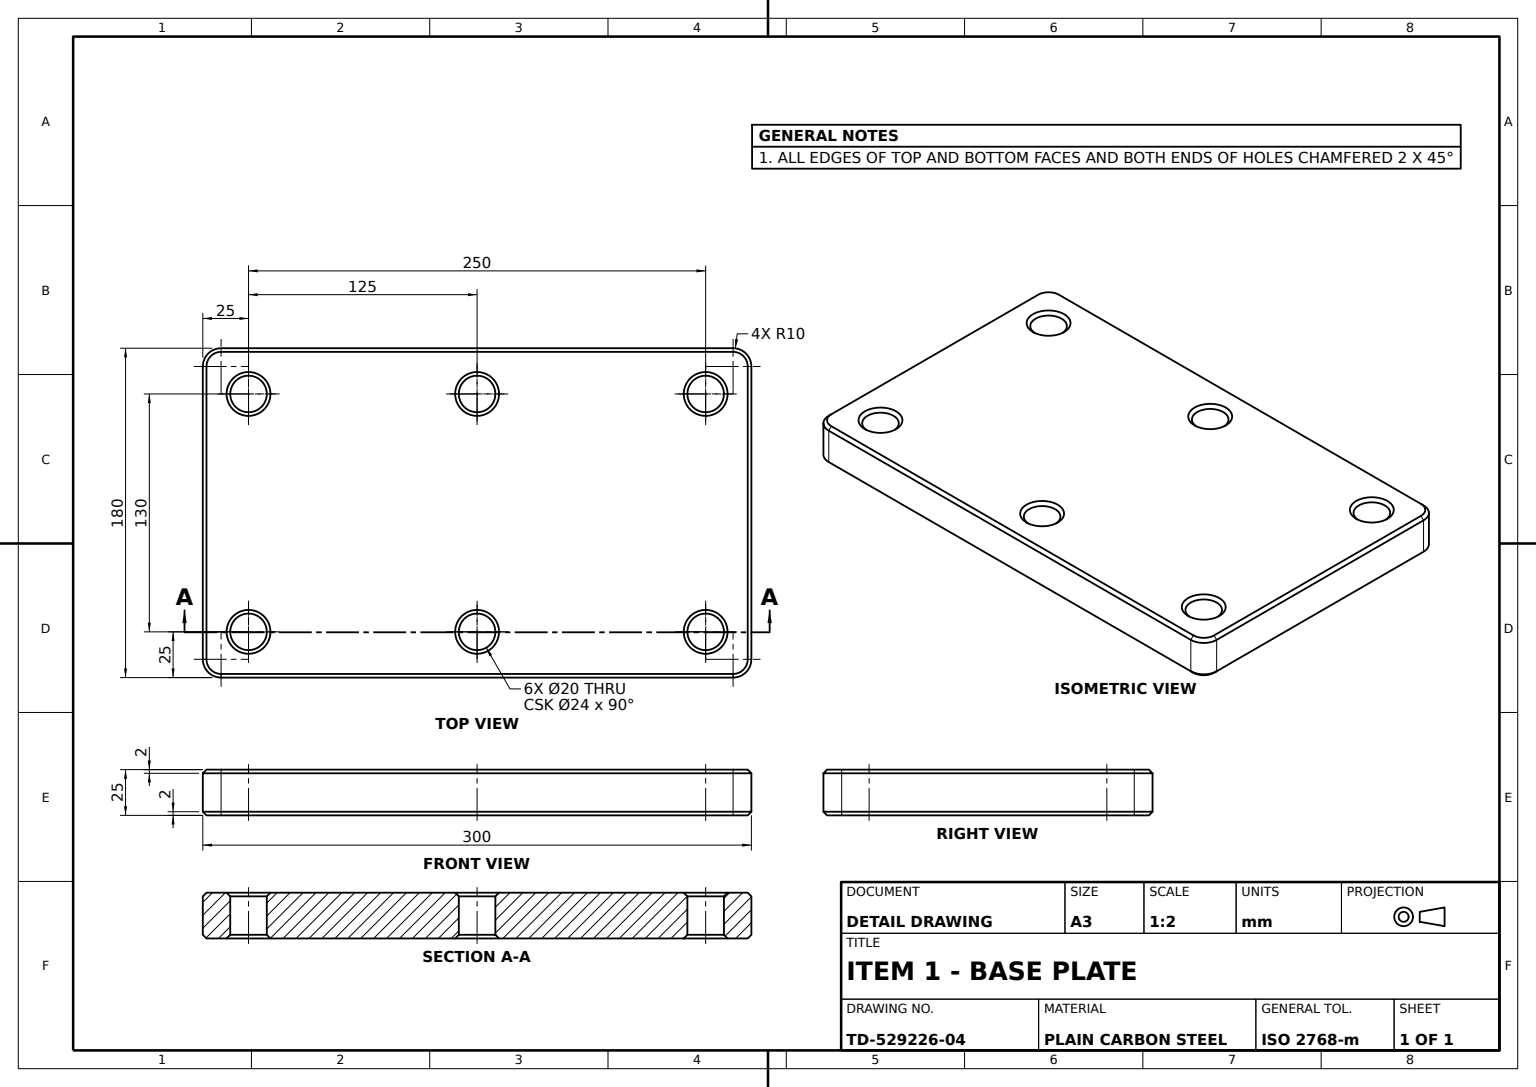
ISO-10303-21;
HEADER;
FILE_DESCRIPTION((''),'2;1');
FILE_NAME('','',(''),(''),'','','');
FILE_SCHEMA(('AUTOMOTIVE_DESIGN'));
ENDSEC;
DATA;
#1=APPLICATION_CONTEXT('');
#2=PRODUCT_CONTEXT('',#1,'mechanical');
#3=PRODUCT('','','',(#2));
#4=PRODUCT_DEFINITION_FORMATION('','',#3);
#5=PRODUCT_DEFINITION_CONTEXT('',#1,'design');
#6=PRODUCT_DEFINITION('','',#4,#5);
#7=PRODUCT_DEFINITION_SHAPE('','',#6);
#8=(LENGTH_UNIT()NAMED_UNIT(*)SI_UNIT(.MILLI.,.METRE.));
#9=(NAMED_UNIT(*)PLANE_ANGLE_UNIT()SI_UNIT($,.RADIAN.));
#10=(NAMED_UNIT(*)SI_UNIT($,.STERADIAN.)SOLID_ANGLE_UNIT());
#11=UNCERTAINTY_MEASURE_WITH_UNIT(LENGTH_MEASURE(1.E-05),#8,'distance_accuracy_value','');
#12=(GEOMETRIC_REPRESENTATION_CONTEXT(3)GLOBAL_UNCERTAINTY_ASSIGNED_CONTEXT((#11))GLOBAL_UNIT_ASSIGNED_CONTEXT((#8,#9,#10))REPRESENTATION_CONTEXT('',''));
#13=CARTESIAN_POINT('',(-150.,23.,-80.));
#14=VERTEX_POINT('',#13);
#15=CARTESIAN_POINT('',(-140.,23.,-90.));
#16=VERTEX_POINT('',#15);
#17=CARTESIAN_POINT('',(-140.,23.,-80.));
#18=DIRECTION('',(0.,-1.,0.));
#19=DIRECTION('',(0.,0.,-1.));
#20=AXIS2_PLACEMENT_3D('',#17,#18,#19);
#21=CIRCLE('',#20,10.);
#22=EDGE_CURVE('',#14,#16,#21,.T.);
#23=ORIENTED_EDGE('',*,*,#22,.T.);
#24=CARTESIAN_POINT('',(-140.,2.,-90.));
#25=VERTEX_POINT('',#24);
#26=CARTESIAN_POINT('',(-140.,25.,-90.));
#27=VECTOR('',#18,1000.);
#28=LINE('',#26,#27);
#29=EDGE_CURVE('',#16,#25,#28,.T.);
#30=ORIENTED_EDGE('',*,*,#29,.T.);
#31=CARTESIAN_POINT('',(-150.,2.,-80.));
#32=VERTEX_POINT('',#31);
#33=CARTESIAN_POINT('',(-140.,2.,-80.));
#34=DIRECTION('',(0.,1.,0.));
#35=AXIS2_PLACEMENT_3D('',#33,#34,#19);
#36=CIRCLE('',#35,10.);
#37=EDGE_CURVE('',#25,#32,#36,.T.);
#38=ORIENTED_EDGE('',*,*,#37,.T.);
#39=CARTESIAN_POINT('',(-150.,25.,-80.));
#40=LINE('',#39,#27);
#41=EDGE_CURVE('',#14,#32,#40,.T.);
#42=ORIENTED_EDGE('',*,*,#41,.F.);
#43=EDGE_LOOP('',(#23,#30,#38,#42));
#44=FACE_OUTER_BOUND('',#43,.T.);
#45=CARTESIAN_POINT('',(-140.,25.,-80.));
#46=AXIS2_PLACEMENT_3D('',#45,#18,#19);
#47=CYLINDRICAL_SURFACE('',#46,10.);
#48=ADVANCED_FACE('',(#44),#47,.T.);
#49=CARTESIAN_POINT('',(0.,2.,-55.));
#50=VERTEX_POINT('',#49);
#51=CARTESIAN_POINT('',(0.,2.,-75.));
#52=VERTEX_POINT('',#51);
#53=CARTESIAN_POINT('',(0.,2.,-65.));
#54=AXIS2_PLACEMENT_3D('',#53,#18,#19);
#55=CIRCLE('',#54,10.);
#56=EDGE_CURVE('',#50,#52,#55,.T.);
#57=ORIENTED_EDGE('',*,*,#56,.F.);
#58=CARTESIAN_POINT('',(0.,0.,-53.));
#59=VERTEX_POINT('',#58);
#60=DIRECTION('',(0.,-0.707106781,0.707106781));
#61=VECTOR('',#60,1000.);
#62=LINE('',#58,#61);
#63=EDGE_CURVE('',#50,#59,#62,.T.);
#64=ORIENTED_EDGE('',*,*,#63,.T.);
#65=CARTESIAN_POINT('',(0.,0.,-77.));
#66=VERTEX_POINT('',#65);
#67=CARTESIAN_POINT('',(0.,0.,-65.));
#68=AXIS2_PLACEMENT_3D('',#67,#34,#19);
#69=CIRCLE('',#68,12.);
#70=EDGE_CURVE('',#66,#59,#69,.T.);
#71=ORIENTED_EDGE('',*,*,#70,.F.);
#72=DIRECTION('',(0.,-0.707106781,-0.707106781));
#73=VECTOR('',#72,1000.);
#74=LINE('',#65,#73);
#75=EDGE_CURVE('',#52,#66,#74,.T.);
#76=ORIENTED_EDGE('',*,*,#75,.F.);
#77=EDGE_LOOP('',(#57,#64,#71,#76));
#78=FACE_OUTER_BOUND('',#77,.T.);
#79=AXIS2_PLACEMENT_3D('',#67,#18,#19);
#80=CONICAL_SURFACE('',#79,12.,0.785398163);
#81=ADVANCED_FACE('',(#78),#80,.F.);
#82=CARTESIAN_POINT('',(-140.,23.,90.));
#83=VERTEX_POINT('',#82);
#84=CARTESIAN_POINT('',(-150.,23.,80.));
#85=VERTEX_POINT('',#84);
#86=CARTESIAN_POINT('',(-140.,23.,80.));
#87=AXIS2_PLACEMENT_3D('',#86,#18,#19);
#88=CIRCLE('',#87,10.);
#89=EDGE_CURVE('',#83,#85,#88,.T.);
#90=ORIENTED_EDGE('',*,*,#89,.F.);
#91=CARTESIAN_POINT('',(-140.,25.,88.));
#92=VERTEX_POINT('',#91);
#93=LINE('',#91,#61);
#94=EDGE_CURVE('',#92,#83,#93,.T.);
#95=ORIENTED_EDGE('',*,*,#94,.F.);
#96=CARTESIAN_POINT('',(-148.,25.,80.));
#97=VERTEX_POINT('',#96);
#98=CARTESIAN_POINT('',(-140.,25.,80.));
#99=AXIS2_PLACEMENT_3D('',#98,#34,#19);
#100=CIRCLE('',#99,8.);
#101=EDGE_CURVE('',#97,#92,#100,.T.);
#102=ORIENTED_EDGE('',*,*,#101,.F.);
#103=DIRECTION('',(-0.707106781,-0.707106781,0.));
#104=VECTOR('',#103,1000.);
#105=LINE('',#96,#104);
#106=EDGE_CURVE('',#97,#85,#105,.T.);
#107=ORIENTED_EDGE('',*,*,#106,.T.);
#108=EDGE_LOOP('',(#90,#95,#102,#107));
#109=FACE_OUTER_BOUND('',#108,.T.);
#110=AXIS2_PLACEMENT_3D('',#98,#18,#19);
#111=CONICAL_SURFACE('',#110,8.,0.785398163);
#112=ADVANCED_FACE('',(#109),#111,.T.);
#113=CARTESIAN_POINT('',(0.,23.,-75.));
#114=VERTEX_POINT('',#113);
#115=CARTESIAN_POINT('',(0.,23.,-55.));
#116=VERTEX_POINT('',#115);
#117=CARTESIAN_POINT('',(0.,23.,-65.));
#118=AXIS2_PLACEMENT_3D('',#117,#34,#19);
#119=CIRCLE('',#118,10.);
#120=EDGE_CURVE('',#114,#116,#119,.T.);
#121=ORIENTED_EDGE('',*,*,#120,.F.);
#122=CARTESIAN_POINT('',(0.,25.,-77.));
#123=VERTEX_POINT('',#122);
#124=DIRECTION('',(0.,0.707106781,-0.707106781));
#125=VECTOR('',#124,1000.);
#126=LINE('',#113,#125);
#127=EDGE_CURVE('',#114,#123,#126,.T.);
#128=ORIENTED_EDGE('',*,*,#127,.T.);
#129=CARTESIAN_POINT('',(0.,25.,-53.));
#130=VERTEX_POINT('',#129);
#131=CARTESIAN_POINT('',(0.,25.,-65.));
#132=AXIS2_PLACEMENT_3D('',#131,#18,#19);
#133=CIRCLE('',#132,12.);
#134=EDGE_CURVE('',#130,#123,#133,.T.);
#135=ORIENTED_EDGE('',*,*,#134,.F.);
#136=DIRECTION('',(0.,0.707106781,0.707106781));
#137=VECTOR('',#136,1000.);
#138=LINE('',#115,#137);
#139=EDGE_CURVE('',#116,#130,#138,.T.);
#140=ORIENTED_EDGE('',*,*,#139,.F.);
#141=EDGE_LOOP('',(#121,#128,#135,#140));
#142=FACE_OUTER_BOUND('',#141,.T.);
#143=DIRECTION('',(0.,0.,1.));
#144=AXIS2_PLACEMENT_3D('',#117,#34,#143);
#145=CONICAL_SURFACE('',#144,10.,0.785398163);
#146=ADVANCED_FACE('',(#142),#145,.F.);
#147=CARTESIAN_POINT('',(-125.,2.,55.));
#148=VERTEX_POINT('',#147);
#149=CARTESIAN_POINT('',(-125.,0.,53.));
#150=VERTEX_POINT('',#149);
#151=LINE('',#149,#73);
#152=EDGE_CURVE('',#148,#150,#151,.T.);
#153=ORIENTED_EDGE('',*,*,#152,.T.);
#154=CARTESIAN_POINT('',(-125.,0.,77.));
#155=VERTEX_POINT('',#154);
#156=CARTESIAN_POINT('',(-125.,0.,65.));
#157=AXIS2_PLACEMENT_3D('',#156,#34,#19);
#158=CIRCLE('',#157,12.);
#159=EDGE_CURVE('',#155,#150,#158,.T.);
#160=ORIENTED_EDGE('',*,*,#159,.F.);
#161=CARTESIAN_POINT('',(-125.,2.,75.));
#162=VERTEX_POINT('',#161);
#163=LINE('',#154,#61);
#164=EDGE_CURVE('',#162,#155,#163,.T.);
#165=ORIENTED_EDGE('',*,*,#164,.F.);
#166=CARTESIAN_POINT('',(-125.,2.,65.));
#167=AXIS2_PLACEMENT_3D('',#166,#18,#19);
#168=CIRCLE('',#167,10.);
#169=EDGE_CURVE('',#148,#162,#168,.T.);
#170=ORIENTED_EDGE('',*,*,#169,.F.);
#171=EDGE_LOOP('',(#153,#160,#165,#170));
#172=FACE_OUTER_BOUND('',#171,.T.);
#173=AXIS2_PLACEMENT_3D('',#156,#18,#19);
#174=CONICAL_SURFACE('',#173,12.,0.785398163);
#175=ADVANCED_FACE('',(#172),#174,.F.);
#176=CARTESIAN_POINT('',(-125.,23.,55.));
#177=VERTEX_POINT('',#176);
#178=CARTESIAN_POINT('',(-125.,25.,55.));
#179=LINE('',#178,#27);
#180=EDGE_CURVE('',#177,#148,#179,.T.);
#181=ORIENTED_EDGE('',*,*,#180,.T.);
#182=ORIENTED_EDGE('',*,*,#169,.T.);
#183=CARTESIAN_POINT('',(-125.,23.,75.));
#184=VERTEX_POINT('',#183);
#185=CARTESIAN_POINT('',(-125.,25.,75.));
#186=LINE('',#185,#27);
#187=EDGE_CURVE('',#184,#162,#186,.T.);
#188=ORIENTED_EDGE('',*,*,#187,.F.);
#189=CARTESIAN_POINT('',(-125.,23.,65.));
#190=AXIS2_PLACEMENT_3D('',#189,#34,#19);
#191=CIRCLE('',#190,10.);
#192=EDGE_CURVE('',#184,#177,#191,.T.);
#193=ORIENTED_EDGE('',*,*,#192,.T.);
#194=EDGE_LOOP('',(#181,#182,#188,#193));
#195=FACE_OUTER_BOUND('',#194,.T.);
#196=CARTESIAN_POINT('',(-125.,25.,65.));
#197=AXIS2_PLACEMENT_3D('',#196,#18,#19);
#198=CYLINDRICAL_SURFACE('',#197,10.);
#199=ADVANCED_FACE('',(#195),#198,.F.);
#200=CARTESIAN_POINT('',(150.,2.,80.));
#201=VERTEX_POINT('',#200);
#202=CARTESIAN_POINT('',(150.,2.,-80.));
#203=VERTEX_POINT('',#202);
#204=VECTOR('',#19,1000.);
#205=LINE('',#202,#204);
#206=EDGE_CURVE('',#201,#203,#205,.T.);
#207=ORIENTED_EDGE('',*,*,#206,.F.);
#208=CARTESIAN_POINT('',(148.,0.,80.));
#209=VERTEX_POINT('',#208);
#210=LINE('',#200,#104);
#211=EDGE_CURVE('',#201,#209,#210,.T.);
#212=ORIENTED_EDGE('',*,*,#211,.T.);
#213=CARTESIAN_POINT('',(148.,0.,-80.));
#214=VERTEX_POINT('',#213);
#215=VECTOR('',#143,1000.);
#216=LINE('',#208,#215);
#217=EDGE_CURVE('',#214,#209,#216,.T.);
#218=ORIENTED_EDGE('',*,*,#217,.F.);
#219=LINE('',#202,#104);
#220=EDGE_CURVE('',#203,#214,#219,.T.);
#221=ORIENTED_EDGE('',*,*,#220,.F.);
#222=EDGE_LOOP('',(#207,#212,#218,#221));
#223=FACE_OUTER_BOUND('',#222,.T.);
#224=DIRECTION('',(0.707106781,-0.707106781,0.));
#225=AXIS2_PLACEMENT_3D('',#202,#224,#143);
#226=PLANE('',#225);
#227=ADVANCED_FACE('',(#223),#226,.T.);
#228=CARTESIAN_POINT('',(140.,0.,-88.));
#229=VERTEX_POINT('',#228);
#230=CARTESIAN_POINT('',(140.,0.,-80.));
#231=AXIS2_PLACEMENT_3D('',#230,#18,#19);
#232=CIRCLE('',#231,8.);
#233=EDGE_CURVE('',#229,#214,#232,.T.);
#234=ORIENTED_EDGE('',*,*,#233,.F.);
#235=CARTESIAN_POINT('',(140.,2.,-90.));
#236=VERTEX_POINT('',#235);
#237=LINE('',#235,#61);
#238=EDGE_CURVE('',#236,#229,#237,.T.);
#239=ORIENTED_EDGE('',*,*,#238,.F.);
#240=CARTESIAN_POINT('',(140.,2.,-80.));
#241=AXIS2_PLACEMENT_3D('',#240,#34,#19);
#242=CIRCLE('',#241,10.);
#243=EDGE_CURVE('',#203,#236,#242,.T.);
#244=ORIENTED_EDGE('',*,*,#243,.F.);
#245=ORIENTED_EDGE('',*,*,#220,.T.);
#246=EDGE_LOOP('',(#234,#239,#244,#245));
#247=FACE_OUTER_BOUND('',#246,.T.);
#248=AXIS2_PLACEMENT_3D('',#240,#34,#143);
#249=CONICAL_SURFACE('',#248,10.,0.785398163);
#250=ADVANCED_FACE('',(#247),#249,.T.);
#251=CARTESIAN_POINT('',(-140.,0.,88.));
#252=VERTEX_POINT('',#251);
#253=CARTESIAN_POINT('',(-140.,2.,90.));
#254=VERTEX_POINT('',#253);
#255=LINE('',#251,#137);
#256=EDGE_CURVE('',#252,#254,#255,.T.);
#257=ORIENTED_EDGE('',*,*,#256,.T.);
#258=CARTESIAN_POINT('',(-150.,2.,80.));
#259=VERTEX_POINT('',#258);
#260=CARTESIAN_POINT('',(-140.,2.,80.));
#261=AXIS2_PLACEMENT_3D('',#260,#34,#19);
#262=CIRCLE('',#261,10.);
#263=EDGE_CURVE('',#259,#254,#262,.T.);
#264=ORIENTED_EDGE('',*,*,#263,.F.);
#265=CARTESIAN_POINT('',(-148.,0.,80.));
#266=VERTEX_POINT('',#265);
#267=DIRECTION('',(-0.707106781,0.707106781,0.));
#268=VECTOR('',#267,1000.);
#269=LINE('',#265,#268);
#270=EDGE_CURVE('',#266,#259,#269,.T.);
#271=ORIENTED_EDGE('',*,*,#270,.F.);
#272=CARTESIAN_POINT('',(-140.,0.,80.));
#273=AXIS2_PLACEMENT_3D('',#272,#18,#19);
#274=CIRCLE('',#273,8.);
#275=EDGE_CURVE('',#252,#266,#274,.T.);
#276=ORIENTED_EDGE('',*,*,#275,.F.);
#277=EDGE_LOOP('',(#257,#264,#271,#276));
#278=FACE_OUTER_BOUND('',#277,.T.);
#279=AXIS2_PLACEMENT_3D('',#260,#34,#143);
#280=CONICAL_SURFACE('',#279,10.,0.785398163);
#281=ADVANCED_FACE('',(#278),#280,.T.);
#282=CARTESIAN_POINT('',(0.,2.,75.));
#283=VERTEX_POINT('',#282);
#284=CARTESIAN_POINT('',(0.,0.,77.));
#285=VERTEX_POINT('',#284);
#286=LINE('',#284,#61);
#287=EDGE_CURVE('',#283,#285,#286,.T.);
#288=ORIENTED_EDGE('',*,*,#287,.T.);
#289=CARTESIAN_POINT('',(0.,0.,53.));
#290=VERTEX_POINT('',#289);
#291=CARTESIAN_POINT('',(0.,0.,65.));
#292=AXIS2_PLACEMENT_3D('',#291,#34,#19);
#293=CIRCLE('',#292,12.);
#294=EDGE_CURVE('',#290,#285,#293,.T.);
#295=ORIENTED_EDGE('',*,*,#294,.F.);
#296=CARTESIAN_POINT('',(0.,2.,55.));
#297=VERTEX_POINT('',#296);
#298=LINE('',#289,#73);
#299=EDGE_CURVE('',#297,#290,#298,.T.);
#300=ORIENTED_EDGE('',*,*,#299,.F.);
#301=CARTESIAN_POINT('',(0.,2.,65.));
#302=AXIS2_PLACEMENT_3D('',#301,#18,#19);
#303=CIRCLE('',#302,10.);
#304=EDGE_CURVE('',#283,#297,#303,.T.);
#305=ORIENTED_EDGE('',*,*,#304,.F.);
#306=EDGE_LOOP('',(#288,#295,#300,#305));
#307=FACE_OUTER_BOUND('',#306,.T.);
#308=AXIS2_PLACEMENT_3D('',#291,#18,#19);
#309=CONICAL_SURFACE('',#308,12.,0.785398163);
#310=ADVANCED_FACE('',(#307),#309,.F.);
#311=CARTESIAN_POINT('',(125.,2.,55.));
#312=VERTEX_POINT('',#311);
#313=CARTESIAN_POINT('',(125.,2.,75.));
#314=VERTEX_POINT('',#313);
#315=CARTESIAN_POINT('',(125.,2.,65.));
#316=AXIS2_PLACEMENT_3D('',#315,#18,#19);
#317=CIRCLE('',#316,10.);
#318=EDGE_CURVE('',#312,#314,#317,.T.);
#319=ORIENTED_EDGE('',*,*,#318,.T.);
#320=CARTESIAN_POINT('',(125.,23.,75.));
#321=VERTEX_POINT('',#320);
#322=CARTESIAN_POINT('',(125.,25.,75.));
#323=LINE('',#322,#27);
#324=EDGE_CURVE('',#321,#314,#323,.T.);
#325=ORIENTED_EDGE('',*,*,#324,.F.);
#326=CARTESIAN_POINT('',(125.,23.,55.));
#327=VERTEX_POINT('',#326);
#328=CARTESIAN_POINT('',(125.,23.,65.));
#329=AXIS2_PLACEMENT_3D('',#328,#34,#19);
#330=CIRCLE('',#329,10.);
#331=EDGE_CURVE('',#321,#327,#330,.T.);
#332=ORIENTED_EDGE('',*,*,#331,.T.);
#333=CARTESIAN_POINT('',(125.,25.,55.));
#334=LINE('',#333,#27);
#335=EDGE_CURVE('',#327,#312,#334,.T.);
#336=ORIENTED_EDGE('',*,*,#335,.T.);
#337=EDGE_LOOP('',(#319,#325,#332,#336));
#338=FACE_OUTER_BOUND('',#337,.T.);
#339=CARTESIAN_POINT('',(125.,25.,65.));
#340=AXIS2_PLACEMENT_3D('',#339,#18,#19);
#341=CYLINDRICAL_SURFACE('',#340,10.);
#342=ADVANCED_FACE('',(#338),#341,.F.);
#343=CARTESIAN_POINT('',(140.,25.,88.));
#344=VERTEX_POINT('',#343);
#345=DIRECTION('',(1.,0.,0.));
#346=VECTOR('',#345,1000.);
#347=LINE('',#343,#346);
#348=EDGE_CURVE('',#92,#344,#347,.T.);
#349=ORIENTED_EDGE('',*,*,#348,.F.);
#350=ORIENTED_EDGE('',*,*,#94,.T.);
#351=CARTESIAN_POINT('',(140.,23.,90.));
#352=VERTEX_POINT('',#351);
#353=DIRECTION('',(-1.,0.,0.));
#354=VECTOR('',#353,1000.);
#355=LINE('',#82,#354);
#356=EDGE_CURVE('',#352,#83,#355,.T.);
#357=ORIENTED_EDGE('',*,*,#356,.F.);
#358=LINE('',#343,#61);
#359=EDGE_CURVE('',#344,#352,#358,.T.);
#360=ORIENTED_EDGE('',*,*,#359,.F.);
#361=EDGE_LOOP('',(#349,#350,#357,#360));
#362=FACE_OUTER_BOUND('',#361,.T.);
#363=AXIS2_PLACEMENT_3D('',#343,#72,#345);
#364=PLANE('',#363);
#365=ADVANCED_FACE('',(#362),#364,.F.);
#366=CARTESIAN_POINT('',(125.,0.,53.));
#367=VERTEX_POINT('',#366);
#368=CARTESIAN_POINT('',(125.,0.,77.));
#369=VERTEX_POINT('',#368);
#370=CARTESIAN_POINT('',(125.,0.,65.));
#371=AXIS2_PLACEMENT_3D('',#370,#34,#19);
#372=CIRCLE('',#371,12.);
#373=EDGE_CURVE('',#367,#369,#372,.T.);
#374=ORIENTED_EDGE('',*,*,#373,.F.);
#375=LINE('',#366,#73);
#376=EDGE_CURVE('',#312,#367,#375,.T.);
#377=ORIENTED_EDGE('',*,*,#376,.F.);
#378=EDGE_CURVE('',#314,#312,#317,.T.);
#379=ORIENTED_EDGE('',*,*,#378,.F.);
#380=LINE('',#368,#61);
#381=EDGE_CURVE('',#314,#369,#380,.T.);
#382=ORIENTED_EDGE('',*,*,#381,.T.);
#383=EDGE_LOOP('',(#374,#377,#379,#382));
#384=FACE_OUTER_BOUND('',#383,.T.);
#385=AXIS2_PLACEMENT_3D('',#370,#18,#19);
#386=CONICAL_SURFACE('',#385,12.,0.785398163);
#387=ADVANCED_FACE('',(#384),#386,.F.);
#388=CARTESIAN_POINT('',(-148.,25.,-80.));
#389=VERTEX_POINT('',#388);
#390=DIRECTION('',(0.707106781,0.707106781,0.));
#391=VECTOR('',#390,1000.);
#392=LINE('',#13,#391);
#393=EDGE_CURVE('',#14,#389,#392,.T.);
#394=ORIENTED_EDGE('',*,*,#393,.T.);
#395=CARTESIAN_POINT('',(-140.,25.,-88.));
#396=VERTEX_POINT('',#395);
#397=AXIS2_PLACEMENT_3D('',#45,#34,#19);
#398=CIRCLE('',#397,8.);
#399=EDGE_CURVE('',#396,#389,#398,.T.);
#400=ORIENTED_EDGE('',*,*,#399,.F.);
#401=LINE('',#15,#137);
#402=EDGE_CURVE('',#16,#396,#401,.T.);
#403=ORIENTED_EDGE('',*,*,#402,.F.);
#404=ORIENTED_EDGE('',*,*,#22,.F.);
#405=EDGE_LOOP('',(#394,#400,#403,#404));
#406=FACE_OUTER_BOUND('',#405,.T.);
#407=CONICAL_SURFACE('',#46,8.,0.785398163);
#408=ADVANCED_FACE('',(#406),#407,.T.);
#409=CARTESIAN_POINT('',(-125.,23.,-55.));
#410=VERTEX_POINT('',#409);
#411=CARTESIAN_POINT('',(-125.,2.,-55.));
#412=VERTEX_POINT('',#411);
#413=CARTESIAN_POINT('',(-125.,25.,-55.));
#414=LINE('',#413,#27);
#415=EDGE_CURVE('',#410,#412,#414,.T.);
#416=ORIENTED_EDGE('',*,*,#415,.T.);
#417=CARTESIAN_POINT('',(-125.,2.,-75.));
#418=VERTEX_POINT('',#417);
#419=CARTESIAN_POINT('',(-125.,2.,-65.));
#420=AXIS2_PLACEMENT_3D('',#419,#18,#19);
#421=CIRCLE('',#420,10.);
#422=EDGE_CURVE('',#412,#418,#421,.T.);
#423=ORIENTED_EDGE('',*,*,#422,.T.);
#424=CARTESIAN_POINT('',(-125.,23.,-75.));
#425=VERTEX_POINT('',#424);
#426=CARTESIAN_POINT('',(-125.,25.,-75.));
#427=LINE('',#426,#27);
#428=EDGE_CURVE('',#425,#418,#427,.T.);
#429=ORIENTED_EDGE('',*,*,#428,.F.);
#430=CARTESIAN_POINT('',(-125.,23.,-65.));
#431=AXIS2_PLACEMENT_3D('',#430,#34,#19);
#432=CIRCLE('',#431,10.);
#433=EDGE_CURVE('',#425,#410,#432,.T.);
#434=ORIENTED_EDGE('',*,*,#433,.T.);
#435=EDGE_LOOP('',(#416,#423,#429,#434));
#436=FACE_OUTER_BOUND('',#435,.T.);
#437=CARTESIAN_POINT('',(-125.,25.,-65.));
#438=AXIS2_PLACEMENT_3D('',#437,#18,#19);
#439=CYLINDRICAL_SURFACE('',#438,10.);
#440=ADVANCED_FACE('',(#436),#439,.F.);
#441=CARTESIAN_POINT('',(0.,25.,-75.));
#442=LINE('',#441,#27);
#443=EDGE_CURVE('',#114,#52,#442,.T.);
#444=ORIENTED_EDGE('',*,*,#443,.F.);
#445=ORIENTED_EDGE('',*,*,#120,.T.);
#446=CARTESIAN_POINT('',(0.,25.,-55.));
#447=LINE('',#446,#27);
#448=EDGE_CURVE('',#116,#50,#447,.T.);
#449=ORIENTED_EDGE('',*,*,#448,.T.);
#450=ORIENTED_EDGE('',*,*,#56,.T.);
#451=EDGE_LOOP('',(#444,#445,#449,#450));
#452=FACE_OUTER_BOUND('',#451,.T.);
#453=CYLINDRICAL_SURFACE('',#132,10.);
#454=ADVANCED_FACE('',(#452),#453,.F.);
#455=CARTESIAN_POINT('',(140.,2.,90.));
#456=VERTEX_POINT('',#455);
#457=LINE('',#455,#346);
#458=EDGE_CURVE('',#254,#456,#457,.T.);
#459=ORIENTED_EDGE('',*,*,#458,.T.);
#460=CARTESIAN_POINT('',(140.,25.,90.));
#461=LINE('',#460,#27);
#462=EDGE_CURVE('',#352,#456,#461,.T.);
#463=ORIENTED_EDGE('',*,*,#462,.F.);
#464=ORIENTED_EDGE('',*,*,#356,.T.);
#465=CARTESIAN_POINT('',(-140.,25.,90.));
#466=LINE('',#465,#27);
#467=EDGE_CURVE('',#83,#254,#466,.T.);
#468=ORIENTED_EDGE('',*,*,#467,.T.);
#469=EDGE_LOOP('',(#459,#463,#464,#468));
#470=FACE_OUTER_BOUND('',#469,.T.);
#471=AXIS2_PLACEMENT_3D('',#465,#19,#353);
#472=PLANE('',#471);
#473=ADVANCED_FACE('',(#470),#472,.F.);
#474=CARTESIAN_POINT('',(-140.,0.,-88.));
#475=VERTEX_POINT('',#474);
#476=LINE('',#228,#346);
#477=EDGE_CURVE('',#475,#229,#476,.T.);
#478=ORIENTED_EDGE('',*,*,#477,.F.);
#479=LINE('',#474,#125);
#480=EDGE_CURVE('',#475,#25,#479,.T.);
#481=ORIENTED_EDGE('',*,*,#480,.T.);
#482=LINE('',#24,#354);
#483=EDGE_CURVE('',#236,#25,#482,.T.);
#484=ORIENTED_EDGE('',*,*,#483,.F.);
#485=ORIENTED_EDGE('',*,*,#238,.T.);
#486=EDGE_LOOP('',(#478,#481,#484,#485));
#487=FACE_OUTER_BOUND('',#486,.T.);
#488=AXIS2_PLACEMENT_3D('',#24,#72,#345);
#489=PLANE('',#488);
#490=ADVANCED_FACE('',(#487),#489,.T.);
#491=CARTESIAN_POINT('',(125.,2.,-75.));
#492=VERTEX_POINT('',#491);
#493=CARTESIAN_POINT('',(125.,0.,-77.));
#494=VERTEX_POINT('',#493);
#495=LINE('',#493,#73);
#496=EDGE_CURVE('',#492,#494,#495,.T.);
#497=ORIENTED_EDGE('',*,*,#496,.T.);
#498=CARTESIAN_POINT('',(125.,0.,-53.));
#499=VERTEX_POINT('',#498);
#500=CARTESIAN_POINT('',(125.,0.,-65.));
#501=AXIS2_PLACEMENT_3D('',#500,#34,#19);
#502=CIRCLE('',#501,12.);
#503=EDGE_CURVE('',#499,#494,#502,.T.);
#504=ORIENTED_EDGE('',*,*,#503,.F.);
#505=CARTESIAN_POINT('',(125.,2.,-55.));
#506=VERTEX_POINT('',#505);
#507=LINE('',#498,#61);
#508=EDGE_CURVE('',#506,#499,#507,.T.);
#509=ORIENTED_EDGE('',*,*,#508,.F.);
#510=CARTESIAN_POINT('',(125.,2.,-65.));
#511=AXIS2_PLACEMENT_3D('',#510,#18,#19);
#512=CIRCLE('',#511,10.);
#513=EDGE_CURVE('',#492,#506,#512,.T.);
#514=ORIENTED_EDGE('',*,*,#513,.F.);
#515=EDGE_LOOP('',(#497,#504,#509,#514));
#516=FACE_OUTER_BOUND('',#515,.T.);
#517=AXIS2_PLACEMENT_3D('',#500,#18,#19);
#518=CONICAL_SURFACE('',#517,12.,0.785398163);
#519=ADVANCED_FACE('',(#516),#518,.F.);
#520=CARTESIAN_POINT('',(150.,23.,-80.));
#521=VERTEX_POINT('',#520);
#522=CARTESIAN_POINT('',(150.,23.,80.));
#523=VERTEX_POINT('',#522);
#524=LINE('',#520,#215);
#525=EDGE_CURVE('',#521,#523,#524,.T.);
#526=ORIENTED_EDGE('',*,*,#525,.T.);
#527=CARTESIAN_POINT('',(150.,25.,80.));
#528=LINE('',#527,#27);
#529=EDGE_CURVE('',#523,#201,#528,.T.);
#530=ORIENTED_EDGE('',*,*,#529,.T.);
#531=ORIENTED_EDGE('',*,*,#206,.T.);
#532=CARTESIAN_POINT('',(150.,25.,-80.));
#533=LINE('',#532,#27);
#534=EDGE_CURVE('',#521,#203,#533,.T.);
#535=ORIENTED_EDGE('',*,*,#534,.F.);
#536=EDGE_LOOP('',(#526,#530,#531,#535));
#537=FACE_OUTER_BOUND('',#536,.T.);
#538=AXIS2_PLACEMENT_3D('',#532,#353,#143);
#539=PLANE('',#538);
#540=ADVANCED_FACE('',(#537),#539,.F.);
#541=CARTESIAN_POINT('',(148.,25.,80.));
#542=VERTEX_POINT('',#541);
#543=VECTOR('',#224,1000.);
#544=LINE('',#541,#543);
#545=EDGE_CURVE('',#542,#523,#544,.T.);
#546=ORIENTED_EDGE('',*,*,#545,.T.);
#547=ORIENTED_EDGE('',*,*,#525,.F.);
#548=CARTESIAN_POINT('',(148.,25.,-80.));
#549=VERTEX_POINT('',#548);
#550=LINE('',#520,#268);
#551=EDGE_CURVE('',#521,#549,#550,.T.);
#552=ORIENTED_EDGE('',*,*,#551,.T.);
#553=LINE('',#548,#204);
#554=EDGE_CURVE('',#542,#549,#553,.T.);
#555=ORIENTED_EDGE('',*,*,#554,.F.);
#556=EDGE_LOOP('',(#546,#547,#552,#555));
#557=FACE_OUTER_BOUND('',#556,.T.);
#558=AXIS2_PLACEMENT_3D('',#548,#103,#19);
#559=PLANE('',#558);
#560=ADVANCED_FACE('',(#557),#559,.F.);
#561=CARTESIAN_POINT('',(140.,23.,-90.));
#562=VERTEX_POINT('',#561);
#563=CARTESIAN_POINT('',(140.,25.,-88.));
#564=VERTEX_POINT('',#563);
#565=LINE('',#561,#137);
#566=EDGE_CURVE('',#562,#564,#565,.T.);
#567=ORIENTED_EDGE('',*,*,#566,.F.);
#568=LINE('',#15,#346);
#569=EDGE_CURVE('',#16,#562,#568,.T.);
#570=ORIENTED_EDGE('',*,*,#569,.F.);
#571=ORIENTED_EDGE('',*,*,#402,.T.);
#572=LINE('',#563,#354);
#573=EDGE_CURVE('',#564,#396,#572,.T.);
#574=ORIENTED_EDGE('',*,*,#573,.F.);
#575=EDGE_LOOP('',(#567,#570,#571,#574));
#576=FACE_OUTER_BOUND('',#575,.T.);
#577=AXIS2_PLACEMENT_3D('',#563,#60,#353);
#578=PLANE('',#577);
#579=ADVANCED_FACE('',(#576),#578,.F.);
#580=CARTESIAN_POINT('',(125.,23.,-75.));
#581=VERTEX_POINT('',#580);
#582=CARTESIAN_POINT('',(125.,25.,-77.));
#583=VERTEX_POINT('',#582);
#584=LINE('',#580,#125);
#585=EDGE_CURVE('',#581,#583,#584,.T.);
#586=ORIENTED_EDGE('',*,*,#585,.F.);
#587=CARTESIAN_POINT('',(125.,23.,-55.));
#588=VERTEX_POINT('',#587);
#589=CARTESIAN_POINT('',(125.,23.,-65.));
#590=AXIS2_PLACEMENT_3D('',#589,#34,#19);
#591=CIRCLE('',#590,10.);
#592=EDGE_CURVE('',#588,#581,#591,.T.);
#593=ORIENTED_EDGE('',*,*,#592,.F.);
#594=CARTESIAN_POINT('',(125.,25.,-53.));
#595=VERTEX_POINT('',#594);
#596=LINE('',#587,#137);
#597=EDGE_CURVE('',#588,#595,#596,.T.);
#598=ORIENTED_EDGE('',*,*,#597,.T.);
#599=CARTESIAN_POINT('',(125.,25.,-65.));
#600=AXIS2_PLACEMENT_3D('',#599,#18,#19);
#601=CIRCLE('',#600,12.);
#602=EDGE_CURVE('',#583,#595,#601,.T.);
#603=ORIENTED_EDGE('',*,*,#602,.F.);
#604=EDGE_LOOP('',(#586,#593,#598,#603));
#605=FACE_OUTER_BOUND('',#604,.T.);
#606=AXIS2_PLACEMENT_3D('',#589,#34,#143);
#607=CONICAL_SURFACE('',#606,10.,0.785398163);
#608=ADVANCED_FACE('',(#605),#607,.F.);
#609=CARTESIAN_POINT('',(-125.,0.,-77.));
#610=VERTEX_POINT('',#609);
#611=LINE('',#609,#73);
#612=EDGE_CURVE('',#418,#610,#611,.T.);
#613=ORIENTED_EDGE('',*,*,#612,.T.);
#614=CARTESIAN_POINT('',(-125.,0.,-53.));
#615=VERTEX_POINT('',#614);
#616=CARTESIAN_POINT('',(-125.,0.,-65.));
#617=AXIS2_PLACEMENT_3D('',#616,#34,#19);
#618=CIRCLE('',#617,12.);
#619=EDGE_CURVE('',#615,#610,#618,.T.);
#620=ORIENTED_EDGE('',*,*,#619,.F.);
#621=LINE('',#614,#61);
#622=EDGE_CURVE('',#412,#615,#621,.T.);
#623=ORIENTED_EDGE('',*,*,#622,.F.);
#624=EDGE_CURVE('',#418,#412,#421,.T.);
#625=ORIENTED_EDGE('',*,*,#624,.F.);
#626=EDGE_LOOP('',(#613,#620,#623,#625));
#627=FACE_OUTER_BOUND('',#626,.T.);
#628=AXIS2_PLACEMENT_3D('',#616,#18,#19);
#629=CONICAL_SURFACE('',#628,12.,0.785398163);
#630=ADVANCED_FACE('',(#627),#629,.F.);
#631=EDGE_CURVE('',#59,#66,#69,.T.);
#632=ORIENTED_EDGE('',*,*,#631,.F.);
#633=ORIENTED_EDGE('',*,*,#63,.F.);
#634=EDGE_CURVE('',#52,#50,#55,.T.);
#635=ORIENTED_EDGE('',*,*,#634,.F.);
#636=ORIENTED_EDGE('',*,*,#75,.T.);
#637=EDGE_LOOP('',(#632,#633,#635,#636));
#638=FACE_OUTER_BOUND('',#637,.T.);
#639=ADVANCED_FACE('',(#638),#80,.F.);
#640=CARTESIAN_POINT('',(125.,25.,53.));
#641=VERTEX_POINT('',#640);
#642=LINE('',#326,#125);
#643=EDGE_CURVE('',#327,#641,#642,.T.);
#644=ORIENTED_EDGE('',*,*,#643,.F.);
#645=ORIENTED_EDGE('',*,*,#331,.F.);
#646=CARTESIAN_POINT('',(125.,25.,77.));
#647=VERTEX_POINT('',#646);
#648=LINE('',#320,#137);
#649=EDGE_CURVE('',#321,#647,#648,.T.);
#650=ORIENTED_EDGE('',*,*,#649,.T.);
#651=CIRCLE('',#340,12.);
#652=EDGE_CURVE('',#641,#647,#651,.T.);
#653=ORIENTED_EDGE('',*,*,#652,.F.);
#654=EDGE_LOOP('',(#644,#645,#650,#653));
#655=FACE_OUTER_BOUND('',#654,.T.);
#656=AXIS2_PLACEMENT_3D('',#328,#34,#143);
#657=CONICAL_SURFACE('',#656,10.,0.785398163);
#658=ADVANCED_FACE('',(#655),#657,.F.);
#659=ORIENTED_EDGE('',*,*,#399,.T.);
#660=LINE('',#388,#215);
#661=EDGE_CURVE('',#389,#97,#660,.T.);
#662=ORIENTED_EDGE('',*,*,#661,.T.);
#663=ORIENTED_EDGE('',*,*,#101,.T.);
#664=ORIENTED_EDGE('',*,*,#348,.T.);
#665=CARTESIAN_POINT('',(140.,25.,80.));
#666=AXIS2_PLACEMENT_3D('',#665,#34,#19);
#667=CIRCLE('',#666,8.);
#668=EDGE_CURVE('',#344,#542,#667,.T.);
#669=ORIENTED_EDGE('',*,*,#668,.T.);
#670=ORIENTED_EDGE('',*,*,#554,.T.);
#671=CARTESIAN_POINT('',(140.,25.,-80.));
#672=AXIS2_PLACEMENT_3D('',#671,#34,#19);
#673=CIRCLE('',#672,8.);
#674=EDGE_CURVE('',#549,#564,#673,.T.);
#675=ORIENTED_EDGE('',*,*,#674,.T.);
#676=ORIENTED_EDGE('',*,*,#573,.T.);
#677=EDGE_LOOP('',(#659,#662,#663,#664,#669,#670,#675,#676));
#678=FACE_OUTER_BOUND('',#677,.T.);
#679=CARTESIAN_POINT('',(-125.,25.,77.));
#680=VERTEX_POINT('',#679);
#681=CARTESIAN_POINT('',(-125.,25.,53.));
#682=VERTEX_POINT('',#681);
#683=CIRCLE('',#197,12.);
#684=EDGE_CURVE('',#680,#682,#683,.T.);
#685=ORIENTED_EDGE('',*,*,#684,.T.);
#686=EDGE_CURVE('',#682,#680,#683,.T.);
#687=ORIENTED_EDGE('',*,*,#686,.T.);
#688=EDGE_LOOP('',(#685,#687));
#689=FACE_BOUND('',#688,.T.);
#690=EDGE_CURVE('',#647,#641,#651,.T.);
#691=ORIENTED_EDGE('',*,*,#690,.T.);
#692=ORIENTED_EDGE('',*,*,#652,.T.);
#693=EDGE_LOOP('',(#691,#692));
#694=FACE_BOUND('',#693,.T.);
#695=CARTESIAN_POINT('',(-125.,25.,-53.));
#696=VERTEX_POINT('',#695);
#697=CARTESIAN_POINT('',(-125.,25.,-77.));
#698=VERTEX_POINT('',#697);
#699=CIRCLE('',#438,12.);
#700=EDGE_CURVE('',#696,#698,#699,.T.);
#701=ORIENTED_EDGE('',*,*,#700,.T.);
#702=EDGE_CURVE('',#698,#696,#699,.T.);
#703=ORIENTED_EDGE('',*,*,#702,.T.);
#704=EDGE_LOOP('',(#701,#703));
#705=FACE_BOUND('',#704,.T.);
#706=CARTESIAN_POINT('',(0.,25.,77.));
#707=VERTEX_POINT('',#706);
#708=CARTESIAN_POINT('',(0.,25.,53.));
#709=VERTEX_POINT('',#708);
#710=CARTESIAN_POINT('',(0.,25.,65.));
#711=AXIS2_PLACEMENT_3D('',#710,#18,#19);
#712=CIRCLE('',#711,12.);
#713=EDGE_CURVE('',#707,#709,#712,.T.);
#714=ORIENTED_EDGE('',*,*,#713,.T.);
#715=EDGE_CURVE('',#709,#707,#712,.T.);
#716=ORIENTED_EDGE('',*,*,#715,.T.);
#717=EDGE_LOOP('',(#714,#716));
#718=FACE_BOUND('',#717,.T.);
#719=ORIENTED_EDGE('',*,*,#134,.T.);
#720=EDGE_CURVE('',#123,#130,#133,.T.);
#721=ORIENTED_EDGE('',*,*,#720,.T.);
#722=EDGE_LOOP('',(#719,#721));
#723=FACE_BOUND('',#722,.T.);
#724=ORIENTED_EDGE('',*,*,#602,.T.);
#725=EDGE_CURVE('',#595,#583,#601,.T.);
#726=ORIENTED_EDGE('',*,*,#725,.T.);
#727=EDGE_LOOP('',(#724,#726));
#728=FACE_BOUND('',#727,.T.);
#729=AXIS2_PLACEMENT_3D('',#671,#18,#19);
#730=PLANE('',#729);
#731=ADVANCED_FACE('',(#678,#689,#694,#705,#718,#723,#728),#730,.F.);
#732=ORIENTED_EDGE('',*,*,#529,.F.);
#733=CARTESIAN_POINT('',(140.,23.,80.));
#734=AXIS2_PLACEMENT_3D('',#733,#18,#19);
#735=CIRCLE('',#734,10.);
#736=EDGE_CURVE('',#523,#352,#735,.T.);
#737=ORIENTED_EDGE('',*,*,#736,.T.);
#738=ORIENTED_EDGE('',*,*,#462,.T.);
#739=CARTESIAN_POINT('',(140.,2.,80.));
#740=AXIS2_PLACEMENT_3D('',#739,#34,#19);
#741=CIRCLE('',#740,10.);
#742=EDGE_CURVE('',#456,#201,#741,.T.);
#743=ORIENTED_EDGE('',*,*,#742,.T.);
#744=EDGE_LOOP('',(#732,#737,#738,#743));
#745=FACE_OUTER_BOUND('',#744,.T.);
#746=AXIS2_PLACEMENT_3D('',#665,#18,#19);
#747=CYLINDRICAL_SURFACE('',#746,10.);
#748=ADVANCED_FACE('',(#745),#747,.T.);
#749=ORIENTED_EDGE('',*,*,#211,.F.);
#750=ORIENTED_EDGE('',*,*,#742,.F.);
#751=CARTESIAN_POINT('',(140.,0.,88.));
#752=VERTEX_POINT('',#751);
#753=LINE('',#455,#73);
#754=EDGE_CURVE('',#456,#752,#753,.T.);
#755=ORIENTED_EDGE('',*,*,#754,.T.);
#756=CARTESIAN_POINT('',(140.,0.,80.));
#757=AXIS2_PLACEMENT_3D('',#756,#18,#19);
#758=CIRCLE('',#757,8.);
#759=EDGE_CURVE('',#209,#752,#758,.T.);
#760=ORIENTED_EDGE('',*,*,#759,.F.);
#761=EDGE_LOOP('',(#749,#750,#755,#760));
#762=FACE_OUTER_BOUND('',#761,.T.);
#763=AXIS2_PLACEMENT_3D('',#739,#34,#143);
#764=CONICAL_SURFACE('',#763,10.,0.785398163);
#765=ADVANCED_FACE('',(#762),#764,.T.);
#766=LINE('',#409,#137);
#767=EDGE_CURVE('',#410,#696,#766,.T.);
#768=ORIENTED_EDGE('',*,*,#767,.F.);
#769=ORIENTED_EDGE('',*,*,#433,.F.);
#770=LINE('',#424,#125);
#771=EDGE_CURVE('',#425,#698,#770,.T.);
#772=ORIENTED_EDGE('',*,*,#771,.T.);
#773=ORIENTED_EDGE('',*,*,#700,.F.);
#774=EDGE_LOOP('',(#768,#769,#772,#773));
#775=FACE_OUTER_BOUND('',#774,.T.);
#776=AXIS2_PLACEMENT_3D('',#430,#34,#143);
#777=CONICAL_SURFACE('',#776,10.,0.785398163);
#778=ADVANCED_FACE('',(#775),#777,.F.);
#779=ORIENTED_EDGE('',*,*,#545,.F.);
#780=ORIENTED_EDGE('',*,*,#668,.F.);
#781=ORIENTED_EDGE('',*,*,#359,.T.);
#782=ORIENTED_EDGE('',*,*,#736,.F.);
#783=EDGE_LOOP('',(#779,#780,#781,#782));
#784=FACE_OUTER_BOUND('',#783,.T.);
#785=CONICAL_SURFACE('',#746,8.,0.785398163);
#786=ADVANCED_FACE('',(#784),#785,.T.);
#787=ORIENTED_EDGE('',*,*,#299,.T.);
#788=EDGE_CURVE('',#285,#290,#293,.T.);
#789=ORIENTED_EDGE('',*,*,#788,.F.);
#790=ORIENTED_EDGE('',*,*,#287,.F.);
#791=EDGE_CURVE('',#297,#283,#303,.T.);
#792=ORIENTED_EDGE('',*,*,#791,.F.);
#793=EDGE_LOOP('',(#787,#789,#790,#792));
#794=FACE_OUTER_BOUND('',#793,.T.);
#795=ADVANCED_FACE('',(#794),#309,.F.);
#796=ORIENTED_EDGE('',*,*,#634,.T.);
#797=ORIENTED_EDGE('',*,*,#448,.F.);
#798=EDGE_CURVE('',#116,#114,#119,.T.);
#799=ORIENTED_EDGE('',*,*,#798,.T.);
#800=ORIENTED_EDGE('',*,*,#443,.T.);
#801=EDGE_LOOP('',(#796,#797,#799,#800));
#802=FACE_OUTER_BOUND('',#801,.T.);
#803=ADVANCED_FACE('',(#802),#453,.F.);
#804=ORIENTED_EDGE('',*,*,#192,.F.);
#805=LINE('',#183,#137);
#806=EDGE_CURVE('',#184,#680,#805,.T.);
#807=ORIENTED_EDGE('',*,*,#806,.T.);
#808=ORIENTED_EDGE('',*,*,#686,.F.);
#809=LINE('',#176,#125);
#810=EDGE_CURVE('',#177,#682,#809,.T.);
#811=ORIENTED_EDGE('',*,*,#810,.F.);
#812=EDGE_LOOP('',(#804,#807,#808,#811));
#813=FACE_OUTER_BOUND('',#812,.T.);
#814=AXIS2_PLACEMENT_3D('',#189,#34,#143);
#815=CONICAL_SURFACE('',#814,10.,0.785398163);
#816=ADVANCED_FACE('',(#813),#815,.F.);
#817=ORIENTED_EDGE('',*,*,#643,.T.);
#818=ORIENTED_EDGE('',*,*,#690,.F.);
#819=ORIENTED_EDGE('',*,*,#649,.F.);
#820=EDGE_CURVE('',#327,#321,#330,.T.);
#821=ORIENTED_EDGE('',*,*,#820,.F.);
#822=EDGE_LOOP('',(#817,#818,#819,#821));
#823=FACE_OUTER_BOUND('',#822,.T.);
#824=ADVANCED_FACE('',(#823),#657,.F.);
#825=ORIENTED_EDGE('',*,*,#187,.T.);
#826=EDGE_CURVE('',#162,#148,#168,.T.);
#827=ORIENTED_EDGE('',*,*,#826,.T.);
#828=ORIENTED_EDGE('',*,*,#180,.F.);
#829=EDGE_CURVE('',#177,#184,#191,.T.);
#830=ORIENTED_EDGE('',*,*,#829,.T.);
#831=EDGE_LOOP('',(#825,#827,#828,#830));
#832=FACE_OUTER_BOUND('',#831,.T.);
#833=ADVANCED_FACE('',(#832),#198,.F.);
#834=ORIENTED_EDGE('',*,*,#139,.T.);
#835=ORIENTED_EDGE('',*,*,#720,.F.);
#836=ORIENTED_EDGE('',*,*,#127,.F.);
#837=ORIENTED_EDGE('',*,*,#798,.F.);
#838=EDGE_LOOP('',(#834,#835,#836,#837));
#839=FACE_OUTER_BOUND('',#838,.T.);
#840=ADVANCED_FACE('',(#839),#145,.F.);
#841=LINE('',#13,#204);
#842=EDGE_CURVE('',#85,#14,#841,.T.);
#843=ORIENTED_EDGE('',*,*,#842,.T.);
#844=ORIENTED_EDGE('',*,*,#41,.T.);
#845=LINE('',#258,#215);
#846=EDGE_CURVE('',#32,#259,#845,.T.);
#847=ORIENTED_EDGE('',*,*,#846,.T.);
#848=CARTESIAN_POINT('',(-150.,25.,80.));
#849=LINE('',#848,#27);
#850=EDGE_CURVE('',#85,#259,#849,.T.);
#851=ORIENTED_EDGE('',*,*,#850,.F.);
#852=EDGE_LOOP('',(#843,#844,#847,#851));
#853=FACE_OUTER_BOUND('',#852,.T.);
#854=AXIS2_PLACEMENT_3D('',#39,#345,#19);
#855=PLANE('',#854);
#856=ADVANCED_FACE('',(#853),#855,.F.);
#857=ORIENTED_EDGE('',*,*,#702,.F.);
#858=ORIENTED_EDGE('',*,*,#771,.F.);
#859=EDGE_CURVE('',#410,#425,#432,.T.);
#860=ORIENTED_EDGE('',*,*,#859,.F.);
#861=ORIENTED_EDGE('',*,*,#767,.T.);
#862=EDGE_LOOP('',(#857,#858,#860,#861));
#863=FACE_OUTER_BOUND('',#862,.T.);
#864=ADVANCED_FACE('',(#863),#777,.F.);
#865=ORIENTED_EDGE('',*,*,#850,.T.);
#866=ORIENTED_EDGE('',*,*,#263,.T.);
#867=ORIENTED_EDGE('',*,*,#467,.F.);
#868=ORIENTED_EDGE('',*,*,#89,.T.);
#869=EDGE_LOOP('',(#865,#866,#867,#868));
#870=FACE_OUTER_BOUND('',#869,.T.);
#871=CYLINDRICAL_SURFACE('',#110,10.);
#872=ADVANCED_FACE('',(#870),#871,.T.);
#873=ORIENTED_EDGE('',*,*,#566,.T.);
#874=ORIENTED_EDGE('',*,*,#674,.F.);
#875=ORIENTED_EDGE('',*,*,#551,.F.);
#876=CARTESIAN_POINT('',(140.,23.,-80.));
#877=AXIS2_PLACEMENT_3D('',#876,#18,#19);
#878=CIRCLE('',#877,10.);
#879=EDGE_CURVE('',#562,#521,#878,.T.);
#880=ORIENTED_EDGE('',*,*,#879,.F.);
#881=EDGE_LOOP('',(#873,#874,#875,#880));
#882=FACE_OUTER_BOUND('',#881,.T.);
#883=CONICAL_SURFACE('',#729,8.,0.785398163);
#884=ADVANCED_FACE('',(#882),#883,.T.);
#885=ORIENTED_EDGE('',*,*,#534,.T.);
#886=ORIENTED_EDGE('',*,*,#243,.T.);
#887=CARTESIAN_POINT('',(140.,25.,-90.));
#888=LINE('',#887,#27);
#889=EDGE_CURVE('',#562,#236,#888,.T.);
#890=ORIENTED_EDGE('',*,*,#889,.F.);
#891=ORIENTED_EDGE('',*,*,#879,.T.);
#892=EDGE_LOOP('',(#885,#886,#890,#891));
#893=FACE_OUTER_BOUND('',#892,.T.);
#894=CYLINDRICAL_SURFACE('',#729,10.);
#895=ADVANCED_FACE('',(#893),#894,.T.);
#896=ORIENTED_EDGE('',*,*,#624,.T.);
#897=ORIENTED_EDGE('',*,*,#415,.F.);
#898=ORIENTED_EDGE('',*,*,#859,.T.);
#899=ORIENTED_EDGE('',*,*,#428,.T.);
#900=EDGE_LOOP('',(#896,#897,#898,#899));
#901=FACE_OUTER_BOUND('',#900,.T.);
#902=ADVANCED_FACE('',(#901),#439,.F.);
#903=EDGE_CURVE('',#494,#499,#502,.T.);
#904=ORIENTED_EDGE('',*,*,#903,.F.);
#905=ORIENTED_EDGE('',*,*,#496,.F.);
#906=EDGE_CURVE('',#506,#492,#512,.T.);
#907=ORIENTED_EDGE('',*,*,#906,.F.);
#908=ORIENTED_EDGE('',*,*,#508,.T.);
#909=EDGE_LOOP('',(#904,#905,#907,#908));
#910=FACE_OUTER_BOUND('',#909,.T.);
#911=ADVANCED_FACE('',(#910),#518,.F.);
#912=CARTESIAN_POINT('',(0.,23.,55.));
#913=VERTEX_POINT('',#912);
#914=LINE('',#912,#125);
#915=EDGE_CURVE('',#913,#709,#914,.T.);
#916=ORIENTED_EDGE('',*,*,#915,.T.);
#917=ORIENTED_EDGE('',*,*,#713,.F.);
#918=CARTESIAN_POINT('',(0.,23.,75.));
#919=VERTEX_POINT('',#918);
#920=LINE('',#918,#137);
#921=EDGE_CURVE('',#919,#707,#920,.T.);
#922=ORIENTED_EDGE('',*,*,#921,.F.);
#923=CARTESIAN_POINT('',(0.,23.,65.));
#924=AXIS2_PLACEMENT_3D('',#923,#34,#19);
#925=CIRCLE('',#924,10.);
#926=EDGE_CURVE('',#913,#919,#925,.T.);
#927=ORIENTED_EDGE('',*,*,#926,.F.);
#928=EDGE_LOOP('',(#916,#917,#922,#927));
#929=FACE_OUTER_BOUND('',#928,.T.);
#930=AXIS2_PLACEMENT_3D('',#923,#34,#143);
#931=CONICAL_SURFACE('',#930,10.,0.785398163);
#932=ADVANCED_FACE('',(#929),#931,.F.);
#933=ORIENTED_EDGE('',*,*,#294,.T.);
#934=ORIENTED_EDGE('',*,*,#788,.T.);
#935=EDGE_LOOP('',(#933,#934));
#936=FACE_BOUND('',#935,.T.);
#937=ORIENTED_EDGE('',*,*,#503,.T.);
#938=ORIENTED_EDGE('',*,*,#903,.T.);
#939=EDGE_LOOP('',(#937,#938));
#940=FACE_BOUND('',#939,.T.);
#941=EDGE_CURVE('',#150,#155,#158,.T.);
#942=ORIENTED_EDGE('',*,*,#941,.T.);
#943=ORIENTED_EDGE('',*,*,#159,.T.);
#944=EDGE_LOOP('',(#942,#943));
#945=FACE_BOUND('',#944,.T.);
#946=ORIENTED_EDGE('',*,*,#619,.T.);
#947=EDGE_CURVE('',#610,#615,#618,.T.);
#948=ORIENTED_EDGE('',*,*,#947,.T.);
#949=EDGE_LOOP('',(#946,#948));
#950=FACE_BOUND('',#949,.T.);
#951=ORIENTED_EDGE('',*,*,#70,.T.);
#952=ORIENTED_EDGE('',*,*,#631,.T.);
#953=EDGE_LOOP('',(#951,#952));
#954=FACE_BOUND('',#953,.T.);
#955=ORIENTED_EDGE('',*,*,#233,.T.);
#956=ORIENTED_EDGE('',*,*,#217,.T.);
#957=ORIENTED_EDGE('',*,*,#759,.T.);
#958=LINE('',#251,#354);
#959=EDGE_CURVE('',#752,#252,#958,.T.);
#960=ORIENTED_EDGE('',*,*,#959,.T.);
#961=ORIENTED_EDGE('',*,*,#275,.T.);
#962=CARTESIAN_POINT('',(-148.,0.,-80.));
#963=VERTEX_POINT('',#962);
#964=LINE('',#962,#204);
#965=EDGE_CURVE('',#266,#963,#964,.T.);
#966=ORIENTED_EDGE('',*,*,#965,.T.);
#967=CARTESIAN_POINT('',(-140.,0.,-80.));
#968=AXIS2_PLACEMENT_3D('',#967,#18,#19);
#969=CIRCLE('',#968,8.);
#970=EDGE_CURVE('',#963,#475,#969,.T.);
#971=ORIENTED_EDGE('',*,*,#970,.T.);
#972=ORIENTED_EDGE('',*,*,#477,.T.);
#973=EDGE_LOOP('',(#955,#956,#957,#960,#961,#966,#971,#972));
#974=FACE_OUTER_BOUND('',#973,.T.);
#975=ORIENTED_EDGE('',*,*,#373,.T.);
#976=EDGE_CURVE('',#369,#367,#372,.T.);
#977=ORIENTED_EDGE('',*,*,#976,.T.);
#978=EDGE_LOOP('',(#975,#977));
#979=FACE_BOUND('',#978,.T.);
#980=PLANE('',#231);
#981=ADVANCED_FACE('',(#936,#940,#945,#950,#954,#974,#979),#980,.T.);
#982=ORIENTED_EDGE('',*,*,#270,.T.);
#983=ORIENTED_EDGE('',*,*,#846,.F.);
#984=LINE('',#962,#268);
#985=EDGE_CURVE('',#963,#32,#984,.T.);
#986=ORIENTED_EDGE('',*,*,#985,.F.);
#987=ORIENTED_EDGE('',*,*,#965,.F.);
#988=EDGE_LOOP('',(#982,#983,#986,#987));
#989=FACE_OUTER_BOUND('',#988,.T.);
#990=AXIS2_PLACEMENT_3D('',#31,#103,#19);
#991=PLANE('',#990);
#992=ADVANCED_FACE('',(#989),#991,.T.);
#993=ORIENTED_EDGE('',*,*,#715,.F.);
#994=ORIENTED_EDGE('',*,*,#915,.F.);
#995=EDGE_CURVE('',#919,#913,#925,.T.);
#996=ORIENTED_EDGE('',*,*,#995,.F.);
#997=ORIENTED_EDGE('',*,*,#921,.T.);
#998=EDGE_LOOP('',(#993,#994,#996,#997));
#999=FACE_OUTER_BOUND('',#998,.T.);
#1000=ADVANCED_FACE('',(#999),#931,.F.);
#1001=ORIENTED_EDGE('',*,*,#29,.F.);
#1002=ORIENTED_EDGE('',*,*,#569,.T.);
#1003=ORIENTED_EDGE('',*,*,#889,.T.);
#1004=ORIENTED_EDGE('',*,*,#483,.T.);
#1005=EDGE_LOOP('',(#1001,#1002,#1003,#1004));
#1006=FACE_OUTER_BOUND('',#1005,.T.);
#1007=AXIS2_PLACEMENT_3D('',#26,#143,#345);
#1008=PLANE('',#1007);
#1009=ADVANCED_FACE('',(#1006),#1008,.F.);
#1010=EDGE_CURVE('',#581,#588,#591,.T.);
#1011=ORIENTED_EDGE('',*,*,#1010,.T.);
#1012=CARTESIAN_POINT('',(125.,25.,-55.));
#1013=LINE('',#1012,#27);
#1014=EDGE_CURVE('',#588,#506,#1013,.T.);
#1015=ORIENTED_EDGE('',*,*,#1014,.T.);
#1016=ORIENTED_EDGE('',*,*,#906,.T.);
#1017=CARTESIAN_POINT('',(125.,25.,-75.));
#1018=LINE('',#1017,#27);
#1019=EDGE_CURVE('',#581,#492,#1018,.T.);
#1020=ORIENTED_EDGE('',*,*,#1019,.F.);
#1021=EDGE_LOOP('',(#1011,#1015,#1016,#1020));
#1022=FACE_OUTER_BOUND('',#1021,.T.);
#1023=CYLINDRICAL_SURFACE('',#600,10.);
#1024=ADVANCED_FACE('',(#1022),#1023,.F.);
#1025=ORIENTED_EDGE('',*,*,#995,.T.);
#1026=CARTESIAN_POINT('',(0.,25.,55.));
#1027=LINE('',#1026,#27);
#1028=EDGE_CURVE('',#913,#297,#1027,.T.);
#1029=ORIENTED_EDGE('',*,*,#1028,.T.);
#1030=ORIENTED_EDGE('',*,*,#791,.T.);
#1031=CARTESIAN_POINT('',(0.,25.,75.));
#1032=LINE('',#1031,#27);
#1033=EDGE_CURVE('',#919,#283,#1032,.T.);
#1034=ORIENTED_EDGE('',*,*,#1033,.F.);
#1035=EDGE_LOOP('',(#1025,#1029,#1030,#1034));
#1036=FACE_OUTER_BOUND('',#1035,.T.);
#1037=CYLINDRICAL_SURFACE('',#711,10.);
#1038=ADVANCED_FACE('',(#1036),#1037,.F.);
#1039=ORIENTED_EDGE('',*,*,#1033,.T.);
#1040=ORIENTED_EDGE('',*,*,#304,.T.);
#1041=ORIENTED_EDGE('',*,*,#1028,.F.);
#1042=ORIENTED_EDGE('',*,*,#926,.T.);
#1043=EDGE_LOOP('',(#1039,#1040,#1041,#1042));
#1044=FACE_OUTER_BOUND('',#1043,.T.);
#1045=ADVANCED_FACE('',(#1044),#1037,.F.);
#1046=ORIENTED_EDGE('',*,*,#684,.F.);
#1047=ORIENTED_EDGE('',*,*,#806,.F.);
#1048=ORIENTED_EDGE('',*,*,#829,.F.);
#1049=ORIENTED_EDGE('',*,*,#810,.T.);
#1050=EDGE_LOOP('',(#1046,#1047,#1048,#1049));
#1051=FACE_OUTER_BOUND('',#1050,.T.);
#1052=ADVANCED_FACE('',(#1051),#815,.F.);
#1053=ORIENTED_EDGE('',*,*,#256,.F.);
#1054=ORIENTED_EDGE('',*,*,#959,.F.);
#1055=ORIENTED_EDGE('',*,*,#754,.F.);
#1056=ORIENTED_EDGE('',*,*,#458,.F.);
#1057=EDGE_LOOP('',(#1053,#1054,#1055,#1056));
#1058=FACE_OUTER_BOUND('',#1057,.T.);
#1059=AXIS2_PLACEMENT_3D('',#253,#60,#353);
#1060=PLANE('',#1059);
#1061=ADVANCED_FACE('',(#1058),#1060,.T.);
#1062=ORIENTED_EDGE('',*,*,#37,.F.);
#1063=ORIENTED_EDGE('',*,*,#480,.F.);
#1064=ORIENTED_EDGE('',*,*,#970,.F.);
#1065=ORIENTED_EDGE('',*,*,#985,.T.);
#1066=EDGE_LOOP('',(#1062,#1063,#1064,#1065));
#1067=FACE_OUTER_BOUND('',#1066,.T.);
#1068=AXIS2_PLACEMENT_3D('',#33,#34,#143);
#1069=CONICAL_SURFACE('',#1068,10.,0.785398163);
#1070=ADVANCED_FACE('',(#1067),#1069,.T.);
#1071=ORIENTED_EDGE('',*,*,#622,.T.);
#1072=ORIENTED_EDGE('',*,*,#947,.F.);
#1073=ORIENTED_EDGE('',*,*,#612,.F.);
#1074=ORIENTED_EDGE('',*,*,#422,.F.);
#1075=EDGE_LOOP('',(#1071,#1072,#1073,#1074));
#1076=FACE_OUTER_BOUND('',#1075,.T.);
#1077=ADVANCED_FACE('',(#1076),#629,.F.);
#1078=ORIENTED_EDGE('',*,*,#585,.T.);
#1079=ORIENTED_EDGE('',*,*,#725,.F.);
#1080=ORIENTED_EDGE('',*,*,#597,.F.);
#1081=ORIENTED_EDGE('',*,*,#1010,.F.);
#1082=EDGE_LOOP('',(#1078,#1079,#1080,#1081));
#1083=FACE_OUTER_BOUND('',#1082,.T.);
#1084=ADVANCED_FACE('',(#1083),#607,.F.);
#1085=ORIENTED_EDGE('',*,*,#324,.T.);
#1086=ORIENTED_EDGE('',*,*,#378,.T.);
#1087=ORIENTED_EDGE('',*,*,#335,.F.);
#1088=ORIENTED_EDGE('',*,*,#820,.T.);
#1089=EDGE_LOOP('',(#1085,#1086,#1087,#1088));
#1090=FACE_OUTER_BOUND('',#1089,.T.);
#1091=ADVANCED_FACE('',(#1090),#341,.F.);
#1092=ORIENTED_EDGE('',*,*,#152,.F.);
#1093=ORIENTED_EDGE('',*,*,#826,.F.);
#1094=ORIENTED_EDGE('',*,*,#164,.T.);
#1095=ORIENTED_EDGE('',*,*,#941,.F.);
#1096=EDGE_LOOP('',(#1092,#1093,#1094,#1095));
#1097=FACE_OUTER_BOUND('',#1096,.T.);
#1098=ADVANCED_FACE('',(#1097),#174,.F.);
#1099=ORIENTED_EDGE('',*,*,#106,.F.);
#1100=ORIENTED_EDGE('',*,*,#661,.F.);
#1101=ORIENTED_EDGE('',*,*,#393,.F.);
#1102=ORIENTED_EDGE('',*,*,#842,.F.);
#1103=EDGE_LOOP('',(#1099,#1100,#1101,#1102));
#1104=FACE_OUTER_BOUND('',#1103,.T.);
#1105=AXIS2_PLACEMENT_3D('',#388,#224,#143);
#1106=PLANE('',#1105);
#1107=ADVANCED_FACE('',(#1104),#1106,.F.);
#1108=ORIENTED_EDGE('',*,*,#318,.F.);
#1109=ORIENTED_EDGE('',*,*,#376,.T.);
#1110=ORIENTED_EDGE('',*,*,#976,.F.);
#1111=ORIENTED_EDGE('',*,*,#381,.F.);
#1112=EDGE_LOOP('',(#1108,#1109,#1110,#1111));
#1113=FACE_OUTER_BOUND('',#1112,.T.);
#1114=ADVANCED_FACE('',(#1113),#386,.F.);
#1115=ORIENTED_EDGE('',*,*,#592,.T.);
#1116=ORIENTED_EDGE('',*,*,#1019,.T.);
#1117=ORIENTED_EDGE('',*,*,#513,.T.);
#1118=ORIENTED_EDGE('',*,*,#1014,.F.);
#1119=EDGE_LOOP('',(#1115,#1116,#1117,#1118));
#1120=FACE_OUTER_BOUND('',#1119,.T.);
#1121=ADVANCED_FACE('',(#1120),#1023,.F.);
#1122=CLOSED_SHELL('',(#48,#81,#112,#146,#175,#199,#227,#250,#281,#310,#342,#365,#387,#408,#440,#454,#473,#490,#519,#540,#560,#579,#608,#630,#639,#658,#731,#748,#765,#778,#786,#795,#803,#816,#824,#833,#840,#856,#864,#872,#884,#895,#902,#911,#932,#981,#992,#1000,#1009,#1024,#1038,#1045,#1052,#1061,#1070,#1077,#1084,#1091,#1098,#1107,#1114,#1121));
#1123=MANIFOLD_SOLID_BREP('',#1122);
#1124=ADVANCED_BREP_SHAPE_REPRESENTATION('',(#1123),#12);
#1125=SHAPE_DEFINITION_REPRESENTATION(#7,#1124);
ENDSEC;
END-ISO-10303-21;
